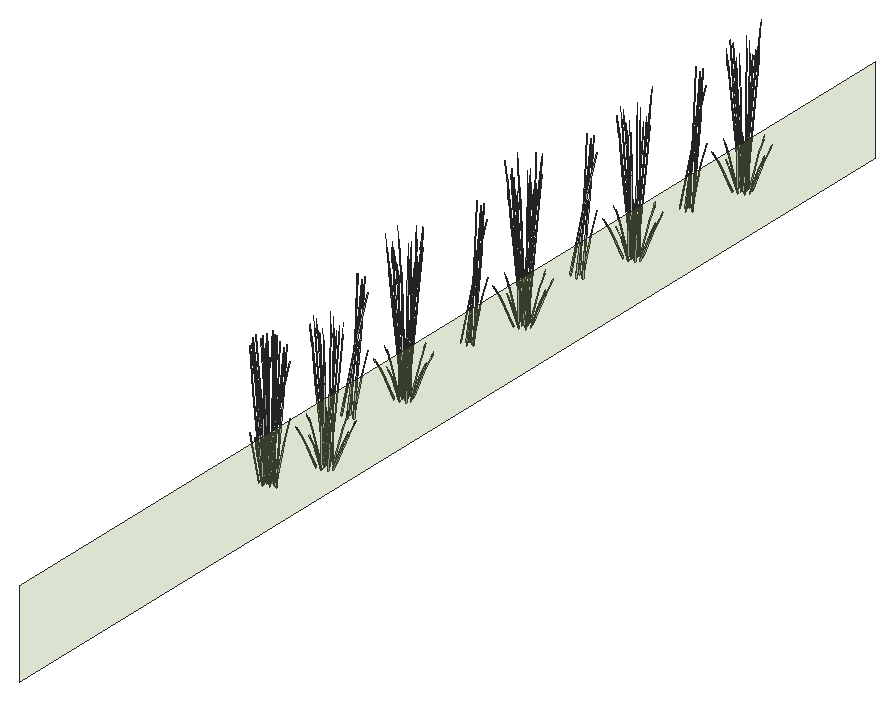
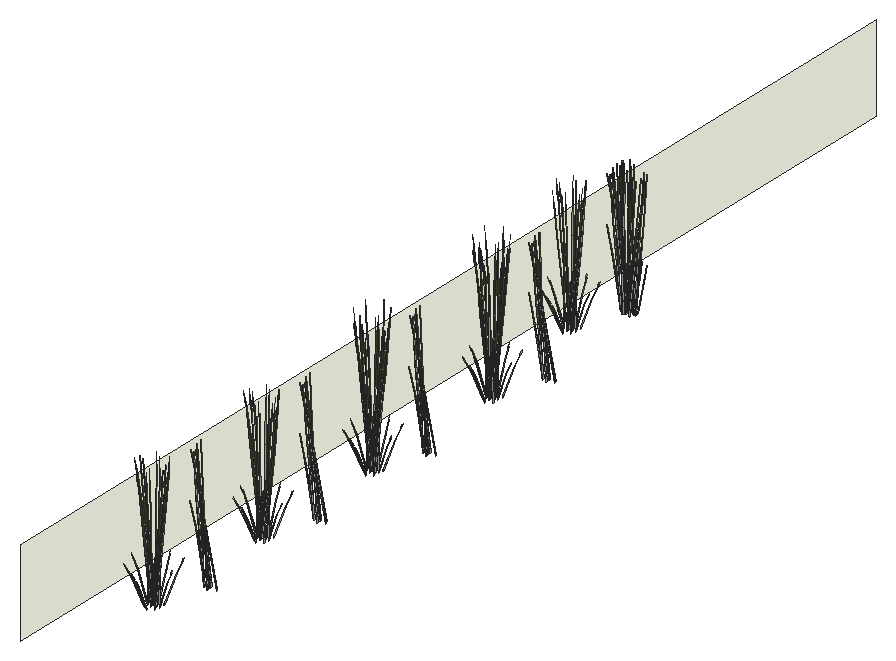
# SketchUp Ruby script. Lengths in inches.
U = 1.inch
M = Sketchup.active_model
def pt(a) = Geom::Point3d.new(a.map { |v| v * U })
def face(e, loops, mat)
  f = e.add_face(loops[0].map { |a| pt(a) })
  loops[1..].each { |l| e.add_face(l.map { |a| pt(a) }).erase! }
  f.material = f.back_material = mat if mat
  f
end
# faces: each face lists its corners as indices into pts; further lists are holes
def faces(e, pts, list, mat = nil) = list.each { |f| face(e, (f[0].is_a?(Array) ? f : [f]).map { |l| l.map { |i| pts[i] } }, mat) }
# xy, xz, yz: faces in a plane at the given z, y or x. An outline is a flat list of corners, or four numbers for a rectangle; further outlines are holes
def ring(l) = l.size == 4 ? [[l[0], l[1]], [l[2], l[1]], [l[2], l[3]], [l[0], l[3]]] : l.each_slice(2).to_a
def flat(e, list, mat, &to3) = list.each { |f| face(e, (f[0].is_a?(Array) ? f : [f]).map { |l| ring(l).map { |u, v| to3.(u, v) } }, mat) }
def xy(e, z, list, mat = nil) = flat(e, list, mat) { |x, y| [x, y, z] }
def xz(e, y, list, mat = nil) = flat(e, list, mat) { |x, z| [x, y, z] }
def yz(e, x, list, mat = nil) = flat(e, list, mat) { |y, z| [x, y, z] }
def lines(e, pts, list) = list.each { |a, b| e.add_line(pt(pts[a]), pt(pts[b])) }
# prism: a flat outline (further loops are holes) pulled along v
def prism(e, loops, v, mat = nil)
  f = face(e, loops, mat); d = Geom::Vector3d.new(v.map { |x| x * U })
  f.pushpull(f.normal.samedirection?(d) ? d.length : -d.length)
end
def box(e, o, s, mat = nil) = prism(e, [[o, [o[0] + s[0], o[1], o[2]], [o[0] + s[0], o[1] + s[1], o[2]], [o[0], o[1] + s[1], o[2]]]], [0, 0, s[2]], mat)
def at(x, y, z, deg = 0) = Geom::Transformation.translation(pt([x, y, z])) * Geom::Transformation.rotation(ORIGIN, Z_AXIS, deg.degrees)
def axes(o, x, y, z) = Geom::Transformation.new([*x, 0, *y, 0, *z, 0, *pt(o).to_a, 1])
def part(name) = M.definitions.add(name)
# library, detail: a bought-in or finely detailed component or shape, given as its bounding box
def library(name, o, s) = part(name).tap { |d| box(d.entities, o, s) }
def detail(e, o, s) = box(e.add_group.entities, o, s)
def put(e, d, t, mat = nil) = e.add_instance(d, t).tap { |i| i.material = mat if mat }
def group(e, t, mat = nil) = e.add_group.tap { |g| g.transformation = t; g.material = mat if mat }.entities
root = M.entities
M.materials.add("Glass_Basic_1").color = [156, 186, 90]
M.materials["Glass_Basic_1"].alpha = 0.25
M.materials.add("LightPink_Translucent").color = [175, 214, 192]
M.materials["LightPink_Translucent"].alpha = 0.75
c1 = part("blade")
p = [[2.15,0.21,22],[0,0.17,0],[0.09,0.45,0],[2.18,0.31,22],[2.29,0.31,22],[0.38,0.45,0],
  [2.48,0.24,33],[2.49,0.24,33],[2.48,0.22,33]]
faces(c1.entities,p,[[0,1,2,3],[4,5,2,3],[6,3,4,7],[8,0,3,6]])
c2 = part("blade with seeds\#1")
put(c2.entities,c1,at(0,0,0))
c3 = part("seeds")
p = [[0.3,-0.1,1.38],[-0.01,-0.03,1.59],[-0.01,-0.03,0.03],[0.14,-0.07,-0.07],[0.29,-0.03,3],[0.15,0.01,3.11]]
faces(c3.entities,p,[[0,1,2,3],[1,0,4,5]],"LightPink_Translucent")
c4 = part("blade with seeds")
put(c4.entities,c1,at(0,0,0))
put(c4.entities,c3,axes([2.4,0.25,30.99],[1.5799,-0.05474,1.17369],[-0.12525,1.92788,0.29478],[-0.07173,-0.02425,1.56792]))
yz(root,510,[[222,138,606,169.19]],"Glass_Basic_1")
put(root,c2,axes([486.97,397.85,138.91],[0.55986,0.18181,-0.23868],[-0.26958,0.38374,-0.41019],[0.01759,0.09422,1.31016]))
put(root,c2,axes([486.97,451.43,138.91],[0.55986,0.18181,-0.23868],[-0.26958,0.38374,-0.41019],[0.01759,0.09422,1.31016]))
put(root,c2,axes([486.97,500.64,138.91],[0.55986,0.18181,-0.23868],[-0.26958,0.38374,-0.41019],[0.01759,0.09422,1.31016]))
put(root,c2,axes([486.97,549.68,138.91],[0.55986,0.18181,-0.23868],[-0.26958,0.38374,-0.41019],[0.01759,0.09422,1.31016]))
put(root,c4,axes([491.15,415.17,138.53],[0.02423,0.07735,1.60472],[-0.13338,0.46528,-0.24515],[-0.15033,0.01361,0.27334]))
put(root,c4,axes([491.15,468.74,138.53],[0.02423,0.07735,1.60472],[-0.13338,0.46528,-0.24515],[-0.15033,0.01361,0.27334]))
put(root,c4,axes([491.15,517.95,138.53],[0.02423,0.07735,1.60472],[-0.13338,0.46528,-0.24515],[-0.15033,0.01361,0.27334]))
put(root,c4,axes([491.15,567,138.53],[0.02423,0.07735,1.60472],[-0.13338,0.46528,-0.24515],[-0.15033,0.01361,0.27334]))
put(root,c2,axes([486.87,398.74,138.51],[0.52192,-0.12929,-0.15749],[0.1834,0.37242,0.00007],[0.05761,-0.01429,1.42656]))
put(root,c2,axes([486.87,452.3125,138.51],[0.52192,-0.12929,-0.15749],[0.1834,0.37242,0.00007],[0.05761,-0.01429,1.42656]))
put(root,c2,axes([486.87,501.52,138.51],[0.52192,-0.12929,-0.15749],[0.1834,0.37242,0.00007],[0.05761,-0.01429,1.42656]))
put(root,c2,axes([486.87,550.57,138.51],[0.52192,-0.12929,-0.15749],[0.1834,0.37242,0.00007],[0.05761,-0.01429,1.42656]))
put(root,c2,axes([486.56,397.45,138.91],[0.50193,-0.25298,-0.23868],[0.33378,0.35745,-0.41019],[0.12384,0.0363,1.31016]))
put(root,c2,axes([486.56,451.03,138.91],[0.50193,-0.25298,-0.23868],[0.33378,0.35745,-0.41019],[0.12384,0.0363,1.31016]))
put(root,c2,axes([486.56,500.24,138.91],[0.50193,-0.25298,-0.23868],[0.33378,0.35745,-0.41019],[0.12384,0.0363,1.31016]))
put(root,c2,axes([486.56,549.28,138.91],[0.50193,-0.25298,-0.23868],[0.33378,0.35745,-0.41019],[0.12384,0.0363,1.31016]))
put(root,c2,axes([488.57,398,138.67],[0.62163,0,0],[0,0.42587,-0.42336],[0,0.097,1.343]))
put(root,c2,axes([488.57,451.58,138.67],[0.62163,0,0],[0,0.42587,-0.42336],[0,0.097,1.343]))
put(root,c2,axes([488.57,500.79,138.67],[0.62163,0,0],[0,0.42587,-0.42336],[0,0.097,1.343]))
put(root,c2,axes([488.57,549.84,138.67],[0.62163,0,0],[0,0.42587,-0.42336],[0,0.097,1.343]))
put(root,c4,axes([491.1875,413.19,138.53],[-0.04449,0.06411,1.60472],[-0.41223,0.1087,-0.24515],[-0.08791,-0.14209,0.27334]))
put(root,c4,axes([491.1875,466.77,138.53],[-0.04449,0.06411,1.60472],[-0.41223,0.1087,-0.24515],[-0.08791,-0.14209,0.27334]))
put(root,c4,axes([491.1875,515.98,138.53],[-0.04449,0.06411,1.60472],[-0.41223,0.1087,-0.24515],[-0.08791,-0.14209,0.27334]))
put(root,c4,axes([491.1875,565.02,138.53],[-0.04449,0.06411,1.60472],[-0.41223,0.1087,-0.24515],[-0.08791,-0.14209,0.27334]))
put(root,c4,axes([491.13,417.22,138.53],[0.06429,0.03482,1.60472],[0.18935,0.43839,-0.24515],[-0.098,0.13291,0.27334]))
put(root,c4,axes([491.13,470.79,138.53],[0.06429,0.03482,1.60472],[0.18935,0.43839,-0.24515],[-0.098,0.13291,0.27334]))
put(root,c4,axes([491.13,520,138.53],[0.06429,0.03482,1.60472],[0.18935,0.43839,-0.24515],[-0.098,0.13291,0.27334]))
put(root,c4,axes([491.13,569.05,138.53],[0.06429,0.03482,1.60472],[0.18935,0.43839,-0.24515],[-0.098,0.13291,0.27334]))
put(root,c2,axes([485.29,397.23,138.02],[-0.48933,0.15256,1.05766],[-0.15575,-0.43772,0.41096],[0.30048,0.00728,1.20297]))
put(root,c2,axes([485.29,450.8,138.02],[-0.48933,0.15256,1.05766],[-0.15575,-0.43772,0.41096],[0.30048,0.00728,1.20297]))
put(root,c2,axes([485.29,500.01,138.02],[-0.48933,0.15256,1.05766],[-0.15575,-0.43772,0.41096],[0.30048,0.00728,1.20297]))
put(root,c2,axes([485.29,549.06,138.02],[-0.48933,0.15256,1.05766],[-0.15575,-0.43772,0.41096],[0.30048,0.00728,1.20297]))
put(root,c2,axes([492.46,355.05,138.76],[-0.31082,0.38183,0],[-0.52,-0.21294,-0.42336],[-0.11843,-0.0485,1.343]))
put(root,c2,axes([487.54,396.55,138.67],[0.31082,-0.38183,0],[0.52,0.21294,-0.42336],[0.11843,0.0485,1.343]))
put(root,c2,axes([487.54,450.125,138.67],[0.31082,-0.38183,0],[0.52,0.21294,-0.42336],[0.11843,0.0485,1.343]))
put(root,c2,axes([487.54,499.33,138.67],[0.31082,-0.38183,0],[0.52,0.21294,-0.42336],[0.11843,0.0485,1.343]))
put(root,c2,axes([487.54,548.38,138.67],[0.31082,-0.38183,0],[0.52,0.21294,-0.42336],[0.11843,0.0485,1.343]))
put(root,c2,axes([491.67,352.18,138.56],[-0.14341,0.31114,-0.03193],[-0.44138,-0.09571,-0.14479],[-0.06702,-0.05089,0.47756]))
put(root,c4,axes([492.71,416.37,139.18],[-0.40128,-0.23189,-0.40713],[0.19312,-0.48183,0.19594],[-0.0925,0,1.30716]))
put(root,c4,axes([492.71,469.94,139.18],[-0.40128,-0.23189,-0.40713],[0.19312,-0.48183,0.19594],[-0.0925,0,1.30716]))
put(root,c4,axes([492.71,519.15,139.18],[-0.40128,-0.23189,-0.40713],[0.19312,-0.48183,0.19594],[-0.0925,0,1.30716]))
put(root,c4,axes([492.71,568.2,139.18],[-0.40128,-0.23189,-0.40713],[0.19312,-0.48183,0.19594],[-0.0925,0,1.30716]))
put(root,c4,axes([492.51,416.15,139.6],[-0.50815,0.05569,-0.26477],[-0.03072,-0.58006,-0.45502],[-0.06769,-0.10214,1.45334]))
put(root,c4,axes([492.51,469.73,139.6],[-0.50815,0.05569,-0.26477],[-0.03072,-0.58006,-0.45502],[-0.06769,-0.10214,1.45334]))
put(root,c4,axes([492.54,417.59,139.02],[-0.27785,-0.33362,-0.2819],[0.27785,-0.33362,0.2819],[-0.08949,0,1.26466]))
put(root,c4,axes([492.54,471.17,139.02],[-0.27785,-0.33362,-0.2819],[0.27785,-0.33362,0.2819],[-0.08949,0,1.26466]))
put(root,c4,axes([492.54,520.375,139.02],[-0.27785,-0.33362,-0.2819],[0.27785,-0.33362,0.2819],[-0.08949,0,1.26466]))
put(root,c4,axes([492.54,569.42,139.02],[-0.27785,-0.33362,-0.2819],[0.27785,-0.33362,0.2819],[-0.08949,0,1.26466]))
put(root,c2,axes([489.35,397.74,138.57],[-0.30821,-0.24366,-0.05322],[0.33756,-0.22326,-0.24131],[0.09565,-0.01572,0.79594]))
put(root,c2,axes([489.35,451.31,138.57],[-0.30821,-0.24366,-0.05322],[0.33756,-0.22326,-0.24131],[0.09565,-0.01572,0.79594]))
put(root,c2,axes([489.35,500.52,138.57],[-0.30821,-0.24366,-0.05322],[0.33756,-0.22326,-0.24131],[0.09565,-0.01572,0.79594]))
put(root,c2,axes([489.35,549.57,138.57],[-0.30821,-0.24366,-0.05322],[0.33756,-0.22326,-0.24131],[0.09565,-0.01572,0.79594]))
put(root,c4,axes([493.05,416.42,139.6],[-0.21249,0.53825,-0.26477],[-0.44849,-0.25917,-0.45502],[-0.11011,0.01692,1.45334]))
put(root,c4,axes([493.05,470,139.6],[-0.21249,0.53825,-0.26477],[-0.44849,-0.25917,-0.45502],[-0.11011,0.01692,1.45334]))
put(root,c2,axes([491.43,353.6,138.76],[-0.62163,0,0],[0,-0.42587,-0.42336],[0,-0.097,1.343]))
put(root,c2,axes([493.44,354.15,139],[-0.50193,0.25298,-0.23868],[-0.33378,-0.35745,-0.41019],[-0.12384,-0.0363,1.31016]))
put(root,c4,axes([491.39,416.23,139.02],[0.11019,-0.44589,-0.2819],[0.38804,0.11227,0.2819],[-0.04475,-0.08989,1.26466]))
put(root,c4,axes([491.39,469.8,139.02],[0.11019,-0.44589,-0.2819],[0.38804,0.11227,0.2819],[-0.04475,-0.08989,1.26466]))
put(root,c4,axes([491.39,519.01,139.02],[0.11019,-0.44589,-0.2819],[0.38804,0.11227,0.2819],[-0.04475,-0.08989,1.26466]))
put(root,c4,axes([491.39,568.0625,139.02],[0.11019,-0.44589,-0.2819],[0.38804,0.11227,0.2819],[-0.04475,-0.08989,1.26466]))
put(root,c2,axes([491.91,353.49,138.72],[-0.46241,0.32036,0.25231],[-0.46269,-0.31699,-0.29936],[-0.01615,-0.09098,1.35263]))
put(root,c2,axes([494,354.27,138.84],[-0.48544,-0.30669,-0.20666],[0.40848,-0.34439,0.45226],[-0.13072,0.03588,1.37996]))
put(root,c4,axes([492.39,415.79,139.18],[-0.02749,-0.519,-0.40713],[0.45634,-0.04694,0.19594],[-0.04625,-0.09291,1.30716]))
put(root,c4,axes([492.39,469.36,139.18],[-0.02749,-0.519,-0.40713],[0.45634,-0.04694,0.19594],[-0.04625,-0.09291,1.30716]))
put(root,c4,axes([492.39,518.57,139.18],[-0.02749,-0.519,-0.40713],[0.45634,-0.04694,0.19594],[-0.04625,-0.09291,1.30716]))
put(root,c4,axes([492.39,567.62,139.18],[-0.02749,-0.519,-0.40713],[0.45634,-0.04694,0.19594],[-0.04625,-0.09291,1.30716]))
put(root,c2,axes([493.16,354.15,138.8125],[0.13176,-0.45152,-0.1922],[0.62475,0.07871,0.4206],[-0.10917,-0.06235,1.28336]))
put(root,c4,axes([493.3,416.33,139.18],[-0.37379,0.28711,-0.40713],[-0.26322,-0.43489,0.19594],[-0.04625,0.09291,1.30716]))
put(root,c4,axes([493.3,469.9,139.18],[-0.37379,0.28711,-0.40713],[-0.26322,-0.43489,0.19594],[-0.04625,0.09291,1.30716]))
put(root,c4,axes([493.3,519.11,139.18],[-0.37379,0.28711,-0.40713],[-0.26322,-0.43489,0.19594],[-0.04625,0.09291,1.30716]))
put(root,c4,axes([493.3,568.16,139.18],[-0.37379,0.28711,-0.40713],[-0.26322,-0.43489,0.19594],[-0.04625,0.09291,1.30716]))
put(root,c2,axes([494.36,355.11,138.61],[-0.30694,-0.38316,-0.04218],[0.52,-0.21294,0.42336],[-0.12814,0.03648,1.34234]))
put(root,c2,axes([488.76,398.06,138.34],[-0.32019,0.04573,1.16148],[-0.05096,-0.36399,0.06648],[0.22426,-0.05509,0.66092]))
put(root,c2,axes([488.76,451.63,138.34],[-0.32019,0.04573,1.16148],[-0.05096,-0.36399,0.06648],[0.22426,-0.05509,0.66092]))
put(root,c2,axes([488.76,500.84,138.34],[-0.32019,0.04573,1.16148],[-0.05096,-0.36399,0.06648],[0.22426,-0.05509,0.66092]))
put(root,c2,axes([488.76,549.89,138.34],[-0.32019,0.04573,1.16148],[-0.05096,-0.36399,0.06648],[0.22426,-0.05509,0.66092]))
put(root,c2,axes([493.02,353.75,139],[-0.55986,-0.18181,-0.23868],[0.26958,-0.38374,-0.41019],[-0.01759,-0.09422,1.31016]))
put(root,c2,axes([494.14,354.09,139],[0.05793,0.43479,-0.23868],[-0.60335,0.02629,-0.41019],[-0.10625,0.05792,1.31016]))
put(root,c2,axes([493.375,351.78,138.56],[-0.34354,0.2186,-0.03193],[-0.31478,-0.23941,-0.14479],[-0.02216,-0.06784,0.47756]))
put(root,c4,axes([494.13,417.12,139.02],[-0.38804,0.11227,-0.2819],[-0.11019,-0.44589,0.2819],[-0.04475,0.08989,1.26466]))
put(root,c4,axes([494.13,470.69,139.02],[-0.38804,0.11227,-0.2819],[-0.11019,-0.44589,0.2819],[-0.04475,0.08989,1.26466]))
put(root,c4,axes([494.13,519.9,139.02],[-0.38804,0.11227,-0.2819],[-0.11019,-0.44589,0.2819],[-0.04475,0.08989,1.26466]))
put(root,c4,axes([494.13,568.95,139.02],[-0.38804,0.11227,-0.2819],[-0.11019,-0.44589,0.2819],[-0.04475,0.08989,1.26466]))
put(root,c4,axes([492.45,415.49,139.6],[-0.29566,-0.48255,-0.26477],[0.41776,-0.32089,-0.45502],[0.04243,-0.11906,1.45334]))
put(root,c4,axes([492.45,469.06,139.6],[-0.29566,-0.48255,-0.26477],[0.41776,-0.32089,-0.45502],[0.04243,-0.11906,1.45334]))
put(root,c2,axes([494.75,355.15,138.76],[0.31082,0.38183,0],[-0.52,0.21294,-0.42336],[-0.11843,0.0485,1.343]))
put(root,c2,axes([493.59,354.72,138.61],[-0.50118,-0.17107,0],[0.2412,-0.35546,0],[0,0,1.33477]))
put(root,c4,axes([493.51,416.02,139.6],[0.29566,0.48255,-0.26477],[-0.41776,0.32089,-0.45502],[-0.04243,0.11906,1.45334]))
put(root,c4,axes([493.51,469.6,139.6],[0.29566,0.48255,-0.26477],[-0.41776,0.32089,-0.45502],[-0.04243,0.11906,1.45334]))
put(root,c4,axes([491.83,414.39,139.02],[0.38804,-0.11227,-0.2819],[0.11019,0.44589,0.2819],[0.04475,-0.08989,1.26466]))
put(root,c4,axes([491.83,467.97,139.02],[0.38804,-0.11227,-0.2819],[0.11019,0.44589,0.2819],[0.04475,-0.08989,1.26466]))
put(root,c4,axes([491.83,517.18,139.02],[0.38804,-0.11227,-0.2819],[0.11019,0.44589,0.2819],[0.04475,-0.08989,1.26466]))
put(root,c4,axes([491.83,566.23,139.02],[0.38804,-0.11227,-0.2819],[0.11019,0.44589,0.2819],[0.04475,-0.08989,1.26466]))
put(root,c4,axes([493.15,413.32,138.53],[-0.07018,0.01212,1.60472],[-0.36652,-0.24435,-0.24515],[0.01847,-0.17356,0.27334]))
put(root,c4,axes([493.15,466.9,138.53],[-0.07018,0.01212,1.60472],[-0.36652,-0.24435,-0.24515],[0.01847,-0.17356,0.27334]))
put(root,c4,axes([493.15,516.11,138.53],[-0.07018,0.01212,1.60472],[-0.36652,-0.24435,-0.24515],[0.01847,-0.17356,0.27334]))
put(root,c4,axes([493.15,565.16,138.53],[-0.07018,0.01212,1.60472],[-0.36652,-0.24435,-0.24515],[0.01847,-0.17356,0.27334]))
put(root,c4,axes([493.08,418.48,138.53],[0.06761,-0.02498,1.60472],[0.39549,0.17324,-0.24515],[0.00569,0.17476,0.27334]))
put(root,c4,axes([493.08,472.05,138.53],[0.06761,-0.02498,1.60472],[0.39549,0.17324,-0.24515],[0.00569,0.17476,0.27334]))
put(root,c4,axes([493.08,521.26,138.53],[0.06761,-0.02498,1.60472],[0.39549,0.17324,-0.24515],[0.00569,0.17476,0.27334]))
put(root,c4,axes([493.08,570.3125,138.53],[0.06761,-0.02498,1.60472],[0.39549,0.17324,-0.24515],[0.00569,0.17476,0.27334]))
put(root,c2,axes([494.37,354.91,138.72],[0.62237,0.12385,0.25231],[-0.1557,0.4427,-0.29936],[-0.10301,0.05541,1.35263]))
put(root,c2,axes([494.12,353.9,138.7],[-0.46241,-0.32797,-0.0503],[0.46269,-0.32817,0],[-0.01615,-0.01145,1.4403]))
put(root,c4,axes([493.78,414.81,138.62],[-0.17829,-0.47044,1.17325],[0.51157,-0.14973,0.45588],[-0.00851,0.28888,1.33444]))
put(root,c4,axes([493.78,468.38,138.62],[-0.17829,-0.47044,1.17325],[0.51157,-0.14973,0.45588],[-0.00851,0.28888,1.33444]))
put(root,c4,axes([493.78,517.59,138.62],[-0.17829,-0.47044,1.17325],[0.51157,-0.14973,0.45588],[-0.00851,0.28888,1.33444]))
put(root,c4,axes([493.78,566.64,138.62],[-0.17829,-0.47044,1.17325],[0.51157,-0.14973,0.45588],[-0.00851,0.28888,1.33444]))
put(root,c2,axes([493.7,354.57,138.62],[-0.1622,-0.32851,0],[0.46318,-0.11504,0],[0,0,1.26638]))
put(root,c2,axes([494.27,353.73,138.69],[0,0.44068,-0.04624],[-0.62163,0,0],[0,0.01385,1.47144]))
put(root,c4,axes([492.66,415.18,139.18],[0.37379,-0.28711,-0.40713],[0.26322,0.43489,0.19594],[0.04625,-0.09291,1.30716]))
put(root,c4,axes([492.66,468.75,139.18],[0.37379,-0.28711,-0.40713],[0.26322,0.43489,0.19594],[0.04625,-0.09291,1.30716]))
put(root,c4,axes([492.66,517.96,139.18],[0.37379,-0.28711,-0.40713],[0.26322,0.43489,0.19594],[0.04625,-0.09291,1.30716]))
put(root,c4,axes([492.66,567.01,139.18],[0.37379,-0.28711,-0.40713],[0.26322,0.43489,0.19594],[0.04625,-0.09291,1.30716]))
put(root,c2,axes([493.96,353.56,138.62],[0,-0.44089,0],[0.62163,0,0],[0,0,1.47217]))
put(root,c2,axes([493.98,354.58,138.69],[0.21614,0.43775,-0.04932],[-0.61757,0.15339,0],[0.00755,0.01529,1.41242]))
put(root,c2,axes([492.69,352.24,138.76],[-0.31082,-0.38183,0],[0.52,-0.21294,-0.42336],[0.11843,-0.0485,1.343]))
put(root,c2,axes([495.76,354.01,138.62],[-0.62132,-0.00305,-0.04082],[0,-0.42587,0.4097],[-0.01953,0.09695,1.29904]))
put(root,c2,axes([494.16,354.73,138.62],[0.50118,0.17107,0],[-0.2412,0.35546,0],[0,0,1.43523]))
put(root,c2,axes([494.38,353.65,138.62],[0.5562,0,0],[0,0.39448,0],[0,0,1.46356]))
put(root,c4,axes([494.57,415.28,139.02],[-0.11019,0.44589,-0.2819],[-0.38804,-0.11227,0.2819],[0.04475,0.08989,1.26466]))
put(root,c4,axes([494.57,468.85,139.02],[-0.11019,0.44589,-0.2819],[-0.38804,-0.11227,0.2819],[0.04475,0.08989,1.26466]))
put(root,c4,axes([494.57,518.0625,139.02],[-0.11019,0.44589,-0.2819],[-0.38804,-0.11227,0.2819],[0.04475,0.08989,1.26466]))
put(root,c4,axes([494.57,567.11,139.02],[-0.11019,0.44589,-0.2819],[-0.38804,-0.11227,0.2819],[0.04475,0.08989,1.26466]))
put(root,c2,axes([493.3,353.29,139],[-0.05793,-0.43479,-0.23868],[0.60335,-0.02629,-0.41019],[0.10625,-0.05792,1.31016]))
put(root,c4,axes([492.92,415.09,139.6],[0.21249,-0.53825,-0.26477],[0.44849,0.25917,-0.45502],[0.11011,-0.01692,1.45334]))
put(root,c4,axes([492.92,468.66,139.6],[0.21249,-0.53825,-0.26477],[0.44849,0.25917,-0.45502],[0.11011,-0.01692,1.45334]))
put(root,c2,axes([494.42,353.64,139],[0.55986,0.18181,-0.23868],[-0.26958,0.38374,-0.41019],[0.01759,0.09422,1.31016]))
put(root,c4,axes([493.42,413.92,139.02],[0.27785,0.33362,-0.2819],[-0.27785,0.33362,0.2819],[0.08949,0,1.26466]))
put(root,c4,axes([493.42,467.49,139.02],[0.27785,0.33362,-0.2819],[-0.27785,0.33362,0.2819],[0.08949,0,1.26466]))
put(root,c4,axes([493.42,516.7,139.02],[0.27785,0.33362,-0.2819],[-0.27785,0.33362,0.2819],[0.08949,0,1.26466]))
put(root,c4,axes([493.42,565.75,139.02],[0.27785,0.33362,-0.2819],[-0.27785,0.33362,0.2819],[0.08949,0,1.26466]))
put(root,c4,axes([493.45,415.35,139.6],[0.50815,-0.05569,-0.26477],[0.03072,0.58006,-0.45502],[0.06769,0.10214,1.45334]))
put(root,c4,axes([493.45,468.93,139.6],[0.50815,-0.05569,-0.26477],[0.03072,0.58006,-0.45502],[0.06769,0.10214,1.45334]))
put(root,c4,axes([493.25,415.14,139.18],[0.40128,0.23189,-0.40713],[-0.19312,0.48183,0.19594],[0.0925,0,1.30716]))
put(root,c4,axes([493.25,468.72,139.18],[0.40128,0.23189,-0.40713],[-0.19312,0.48183,0.19594],[0.0925,0,1.30716]))
put(root,c4,axes([493.25,517.93,139.18],[0.40128,0.23189,-0.40713],[-0.19312,0.48183,0.19594],[0.0925,0,1.30716]))
put(root,c4,axes([493.25,566.98,139.18],[0.40128,0.23189,-0.40713],[-0.19312,0.48183,0.19594],[0.0925,0,1.30716]))
put(root,c4,axes([498.59,370.96,138.625],[0.02423,0.07735,1.60472],[-0.13338,0.46528,-0.24515],[-0.15033,0.01361,0.27334]))
put(root,c2,axes([494.31,354.53,138.61],[0.52192,-0.12929,-0.15749],[0.1834,0.37242,0.00007],[0.05761,-0.01429,1.42656]))
put(root,c2,axes([494,353.24,139],[0.50193,-0.25298,-0.23868],[0.33378,0.35745,-0.41019],[0.12384,0.0363,1.31016]))
put(root,c2,axes([496.01,353.79,138.76],[0.62163,0,0],[0,0.42587,-0.42336],[0,0.097,1.343]))
put(root,c4,axes([494.76,417.47,138.53],[0.03508,-0.07154,1.60472],[0.39195,-0.18375,-0.24515],[0.10636,0.12396,0.27334]))
put(root,c4,axes([494.76,471.04,138.53],[0.03508,-0.07154,1.60472],[0.39195,-0.18375,-0.24515],[0.10636,0.12396,0.27334]))
put(root,c4,axes([494.76,520.25,138.53],[0.03508,-0.07154,1.60472],[0.39195,-0.18375,-0.24515],[0.10636,0.12396,0.27334]))
put(root,c4,axes([494.76,569.3,138.53],[0.03508,-0.07154,1.60472],[0.39195,-0.18375,-0.24515],[0.10636,0.12396,0.27334]))
put(root,c4,axes([498.63,368.98,138.625],[-0.04449,0.06411,1.60472],[-0.41223,0.1087,-0.24515],[-0.08791,-0.14209,0.27334]))
put(root,c4,axes([498.57,373.01,138.625],[0.06429,0.03482,1.60472],[0.18935,0.43839,-0.24515],[-0.098,0.13291,0.27334]))
put(root,c4,axes([494.98,414.07,138.53],[-0.05867,-0.0463,1.60472],[-0.12648,-0.46786,-0.24515],[0.11506,-0.11302,0.27334]))
put(root,c4,axes([494.98,467.65,138.53],[-0.05867,-0.0463,1.60472],[-0.12648,-0.46786,-0.24515],[0.11506,-0.11302,0.27334]))
put(root,c4,axes([494.98,516.86,138.53],[-0.05867,-0.0463,1.60472],[-0.12648,-0.46786,-0.24515],[0.11506,-0.11302,0.27334]))
put(root,c4,axes([494.98,565.9,138.53],[-0.05867,-0.0463,1.60472],[-0.12648,-0.46786,-0.24515],[0.11506,-0.11302,0.27334]))
put(root,c2,axes([492.73,353.01,138.12],[-0.48933,0.15256,1.05766],[-0.15575,-0.43772,0.41096],[0.30048,0.00728,1.20297]))
put(root,c2,axes([494.98,352.34,138.76],[0.31082,-0.38183,0],[0.52,0.21294,-0.42336],[0.11843,0.0485,1.343]))
put(root,c4,axes([500.16,372.15,139.28],[-0.40128,-0.23189,-0.40713],[0.19312,-0.48183,0.19594],[-0.0925,0,1.30716]))
put(root,c4,axes([499.98,373.38,139.11],[-0.27785,-0.33362,-0.2819],[0.27785,-0.33362,0.2819],[-0.08949,0,1.26466]))
put(root,c2,axes([496.79,353.52,138.67],[-0.30821,-0.24366,-0.05322],[0.33756,-0.22326,-0.24131],[0.09565,-0.01572,0.79594]))
put(root,c4,axes([498.83,372.02,139.11],[0.11019,-0.44589,-0.2819],[0.38804,0.11227,0.2819],[-0.04475,-0.08989,1.26466]))
put(root,c4,axes([495.53,415.51,138.53],[-0.01605,-0.08017,1.60472],[0.18061,-0.44332,-0.24515],[0.15065,0.00744,0.27334]))
put(root,c4,axes([495.53,469.08,138.53],[-0.01605,-0.08017,1.60472],[0.18061,-0.44332,-0.24515],[0.15065,0.00744,0.27334]))
put(root,c4,axes([495.53,518.29,138.53],[-0.01605,-0.08017,1.60472],[0.18061,-0.44332,-0.24515],[0.15065,0.00744,0.27334]))
put(root,c4,axes([495.53,567.34,138.53],[-0.01605,-0.08017,1.60472],[0.18061,-0.44332,-0.24515],[0.15065,0.00744,0.27334]))
put(root,c4,axes([499.83,371.58,139.28],[-0.02749,-0.519,-0.40713],[0.45634,-0.04694,0.19594],[-0.04625,-0.09291,1.30716]))
put(root,c4,axes([500.75,372.12,139.28],[-0.37379,0.28711,-0.40713],[-0.26322,-0.43489,0.19594],[-0.04625,0.09291,1.30716]))
put(root,c2,axes([496.21,353.85,138.4375],[-0.32019,0.04573,1.16148],[-0.05096,-0.36399,0.06648],[0.22426,-0.05509,0.66092]))
put(root,c4,axes([501.58,372.9,139.11],[-0.38804,0.11227,-0.2819],[-0.11019,-0.44589,0.2819],[-0.04475,0.08989,1.26466]))
put(root,c4,axes([499.27,370.18,139.11],[0.38804,-0.11227,-0.2819],[0.11019,0.44589,0.2819],[0.04475,-0.08989,1.26466]))
put(root,c4,axes([500.59,369.11,138.625],[-0.07018,0.01212,1.60472],[-0.36652,-0.24435,-0.24515],[0.01847,-0.17356,0.27334]))
put(root,c4,axes([500.53,374.27,138.625],[0.06761,-0.02498,1.60472],[0.39549,0.17324,-0.24515],[0.00569,0.17476,0.27334]))
put(root,c4,axes([500.1,370.97,139.28],[0.37379,-0.28711,-0.40713],[0.26322,0.43489,0.19594],[0.04625,-0.09291,1.30716]))
put(root,c4,axes([502.02,371.07,139.11],[-0.11019,0.44589,-0.2819],[-0.38804,-0.11227,0.2819],[0.04475,0.08989,1.26466]))
put(root,c4,axes([500.86,369.7,139.11],[0.27785,0.33362,-0.2819],[-0.27785,0.33362,0.2819],[0.08949,0,1.26466]))
put(root,c4,axes([500.69,370.93,139.28],[0.40128,0.23189,-0.40713],[-0.19312,0.48183,0.19594],[0.0925,0,1.30716]))
put(root,c4,axes([502.21,373.26,138.625],[0.03508,-0.07154,1.60472],[0.39195,-0.18375,-0.24515],[0.10636,0.12396,0.27334]))
put(root,c4,axes([502.42,369.86,138.625],[-0.05867,-0.0463,1.60472],[-0.12648,-0.46786,-0.24515],[0.11506,-0.11302,0.27334]))
put(root,c4,axes([502.97,371.29,138.625],[-0.01605,-0.08017,1.60472],[0.18061,-0.44332,-0.24515],[0.15065,0.00744,0.27334]))
